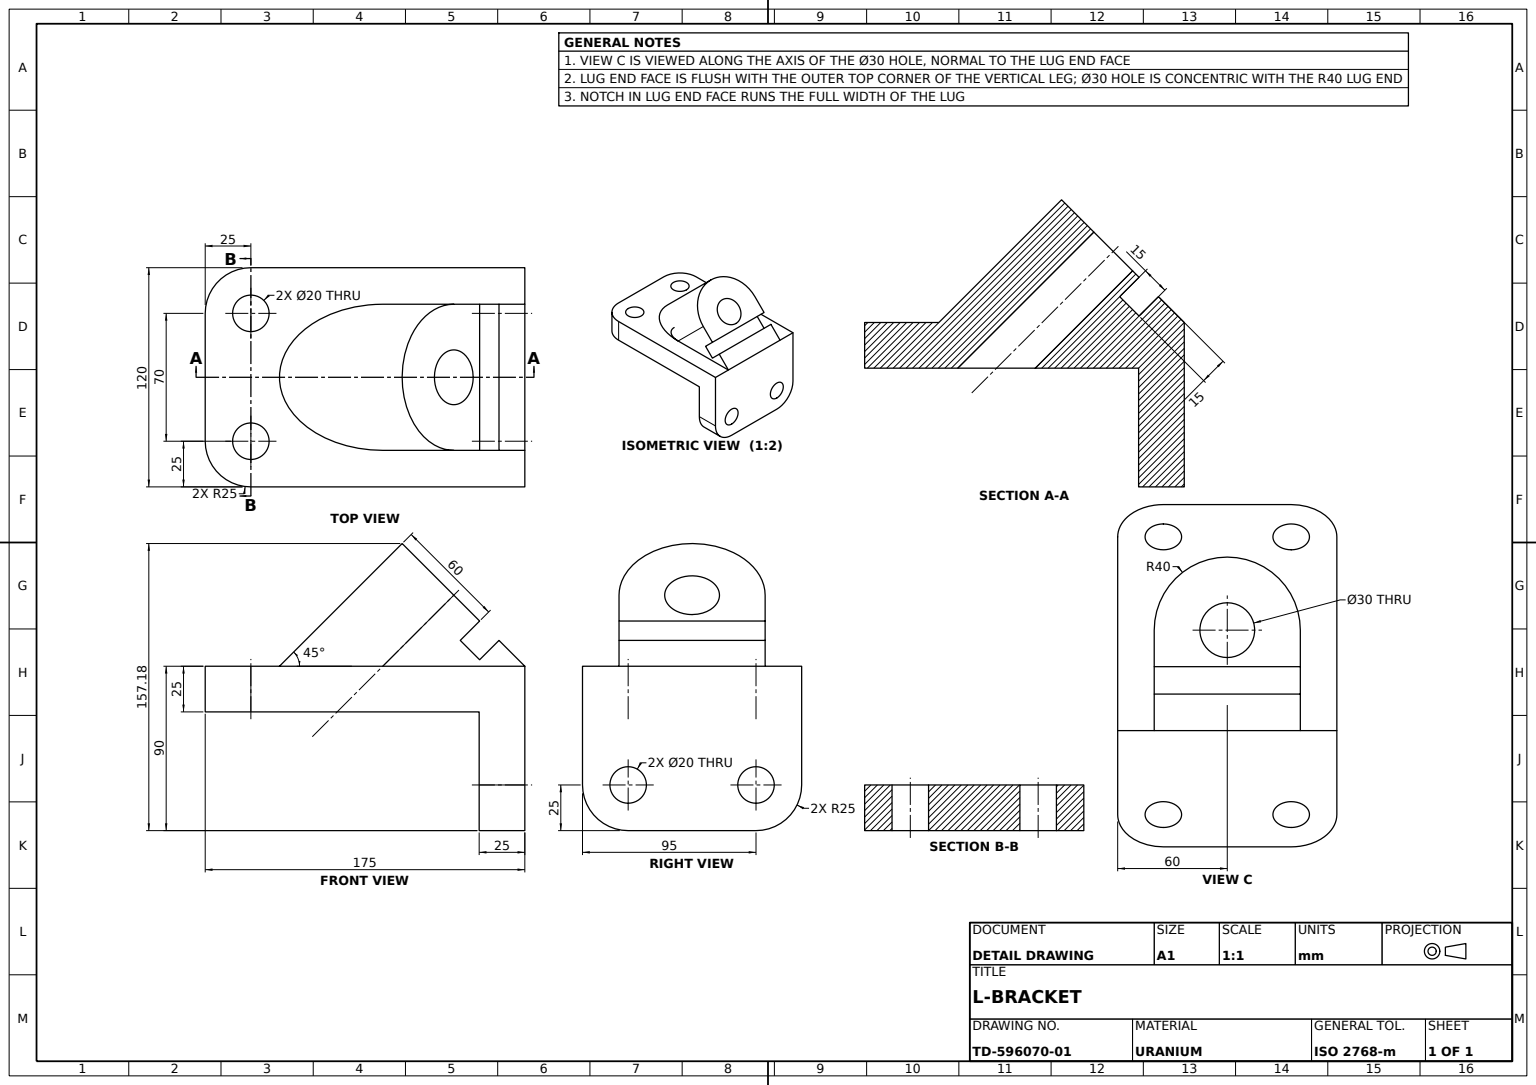
ISO-10303-21;
HEADER;
FILE_DESCRIPTION((''),'2;1');
FILE_NAME('','',(''),(''),'','','');
FILE_SCHEMA(('AUTOMOTIVE_DESIGN'));
ENDSEC;
DATA;
#1=APPLICATION_CONTEXT('');
#2=PRODUCT_CONTEXT('',#1,'mechanical');
#3=PRODUCT('','','',(#2));
#4=PRODUCT_DEFINITION_FORMATION('','',#3);
#5=PRODUCT_DEFINITION_CONTEXT('',#1,'design');
#6=PRODUCT_DEFINITION('','',#4,#5);
#7=PRODUCT_DEFINITION_SHAPE('','',#6);
#8=(LENGTH_UNIT()NAMED_UNIT(*)SI_UNIT(.MILLI.,.METRE.));
#9=(NAMED_UNIT(*)PLANE_ANGLE_UNIT()SI_UNIT($,.RADIAN.));
#10=(NAMED_UNIT(*)SI_UNIT($,.STERADIAN.)SOLID_ANGLE_UNIT());
#11=UNCERTAINTY_MEASURE_WITH_UNIT(LENGTH_MEASURE(0.005),#8,'distance_accuracy_value','');
#12=(GEOMETRIC_REPRESENTATION_CONTEXT(3)GLOBAL_UNCERTAINTY_ASSIGNED_CONTEXT((#11))GLOBAL_UNIT_ASSIGNED_CONTEXT((#8,#9,#10))REPRESENTATION_CONTEXT('',''));
#13=CARTESIAN_POINT('',(-81.568542,0.,-25.));
#14=VERTEX_POINT('',#13);
#15=CARTESIAN_POINT('',(-102.781746,0.,-25.));
#16=DIRECTION('',(0.,0.,1.));
#17=DIRECTION('',(1.,0.,0.));
#18=AXIS2_PLACEMENT_3D('',#15,#16,#17);
#19=ELLIPSE('',#18,21.213203,15.);
#20=EDGE_CURVE('',#14,#14,#19,.T.);
#21=ORIENTED_EDGE('',*,*,#20,.T.);
#22=EDGE_LOOP('',(#21));
#23=FACE_BOUND('',#22,.T.);
#24=CARTESIAN_POINT('',(-140.,-35.,-25.));
#25=VERTEX_POINT('',#24);
#26=CARTESIAN_POINT('',(-150.,-35.,-25.));
#27=AXIS2_PLACEMENT_3D('',#26,#16,#17);
#28=CIRCLE('',#27,10.);
#29=EDGE_CURVE('',#25,#25,#28,.T.);
#30=ORIENTED_EDGE('',*,*,#29,.T.);
#31=EDGE_LOOP('',(#30));
#32=FACE_BOUND('',#31,.T.);
#33=CARTESIAN_POINT('',(-175.,-35.,-25.));
#34=VERTEX_POINT('',#33);
#35=CARTESIAN_POINT('',(-175.,35.,-25.));
#36=VERTEX_POINT('',#35);
#37=CARTESIAN_POINT('',(-175.,0.,-25.));
#38=DIRECTION('',(0.,1.,0.));
#39=VECTOR('',#38,1000.);
#40=LINE('',#37,#39);
#41=EDGE_CURVE('',#34,#36,#40,.T.);
#42=ORIENTED_EDGE('',*,*,#41,.T.);
#43=CARTESIAN_POINT('',(-150.,60.,-25.));
#44=VERTEX_POINT('',#43);
#45=CARTESIAN_POINT('',(-150.,35.,-25.));
#46=AXIS2_PLACEMENT_3D('',#45,#16,#17);
#47=CIRCLE('',#46,25.);
#48=EDGE_CURVE('',#44,#36,#47,.T.);
#49=ORIENTED_EDGE('',*,*,#48,.F.);
#50=CARTESIAN_POINT('',(-25.,60.,-25.));
#51=VERTEX_POINT('',#50);
#52=CARTESIAN_POINT('',(0.,60.,-25.));
#53=VECTOR('',#17,1000.);
#54=LINE('',#52,#53);
#55=EDGE_CURVE('',#44,#51,#54,.T.);
#56=ORIENTED_EDGE('',*,*,#55,.T.);
#57=CARTESIAN_POINT('',(-25.,-60.,-25.));
#58=VERTEX_POINT('',#57);
#59=CARTESIAN_POINT('',(-25.,0.,-25.));
#60=LINE('',#59,#39);
#61=EDGE_CURVE('',#58,#51,#60,.T.);
#62=ORIENTED_EDGE('',*,*,#61,.F.);
#63=CARTESIAN_POINT('',(-150.,-60.,-25.));
#64=VERTEX_POINT('',#63);
#65=CARTESIAN_POINT('',(0.,-60.,-25.));
#66=LINE('',#65,#53);
#67=EDGE_CURVE('',#64,#58,#66,.T.);
#68=ORIENTED_EDGE('',*,*,#67,.F.);
#69=CIRCLE('',#27,25.);
#70=EDGE_CURVE('',#34,#64,#69,.T.);
#71=ORIENTED_EDGE('',*,*,#70,.F.);
#72=EDGE_LOOP('',(#42,#49,#56,#62,#68,#71));
#73=FACE_BOUND('',#72,.T.);
#74=CARTESIAN_POINT('',(-140.,35.,-25.));
#75=VERTEX_POINT('',#74);
#76=CIRCLE('',#46,10.);
#77=EDGE_CURVE('',#75,#75,#76,.T.);
#78=ORIENTED_EDGE('',*,*,#77,.T.);
#79=EDGE_LOOP('',(#78));
#80=FACE_BOUND('',#79,.T.);
#81=AXIS2_PLACEMENT_3D('',#37,#16,#17);
#82=PLANE('',#81);
#83=ADVANCED_FACE('',(#23,#32,#73,#80),#82,.F.);
#84=ORIENTED_EDGE('',*,*,#20,.F.);
#85=EDGE_LOOP('',(#84));
#86=FACE_BOUND('',#85,.T.);
#87=CARTESIAN_POINT('',(-28.284271,0.,28.284271));
#88=VERTEX_POINT('',#87);
#89=CARTESIAN_POINT('',(-38.890873,0.,38.890873));
#90=DIRECTION('',(0.707106781,0.,0.707106781));
#91=DIRECTION('',(0.707106781,0.,-0.707106781));
#92=AXIS2_PLACEMENT_3D('',#89,#90,#91);
#93=CIRCLE('',#92,15.);
#94=EDGE_CURVE('',#88,#88,#93,.T.);
#95=ORIENTED_EDGE('',*,*,#94,.T.);
#96=EDGE_LOOP('',(#95));
#97=FACE_BOUND('',#96,.T.);
#98=CARTESIAN_POINT('',(-116.261028,0.,-38.479282));
#99=AXIS2_PLACEMENT_3D('',#98,#90,#38);
#100=CYLINDRICAL_SURFACE('',#99,15.);
#101=ADVANCED_FACE('',(#86,#97),#100,.F.);
#102=CARTESIAN_POINT('',(-38.890873,40.,38.890873));
#103=VERTEX_POINT('',#102);
#104=CARTESIAN_POINT('',(-24.748737,40.,24.748737));
#105=VERTEX_POINT('',#104);
#106=VECTOR('',#91,1000.);
#107=LINE('',#102,#106);
#108=EDGE_CURVE('',#103,#105,#107,.T.);
#109=ORIENTED_EDGE('',*,*,#108,.T.);
#110=CARTESIAN_POINT('',(-35.355339,40.,14.142136));
#111=VERTEX_POINT('',#110);
#112=DIRECTION('',(-0.707106781,0.,-0.707106781));
#113=VECTOR('',#112,1000.);
#114=LINE('',#104,#113);
#115=EDGE_CURVE('',#105,#111,#114,.T.);
#116=ORIENTED_EDGE('',*,*,#115,.T.);
#117=CARTESIAN_POINT('',(-24.748737,40.,3.535534));
#118=VERTEX_POINT('',#117);
#119=CARTESIAN_POINT('',(-10.606602,40.,-10.606602));
#120=DIRECTION('',(-0.707106781,0.,0.707106781));
#121=VECTOR('',#120,1000.);
#122=LINE('',#119,#121);
#123=EDGE_CURVE('',#118,#111,#122,.T.);
#124=ORIENTED_EDGE('',*,*,#123,.F.);
#125=CARTESIAN_POINT('',(-14.142136,40.,14.142136));
#126=VERTEX_POINT('',#125);
#127=LINE('',#125,#113);
#128=EDGE_CURVE('',#126,#118,#127,.T.);
#129=ORIENTED_EDGE('',*,*,#128,.F.);
#130=CARTESIAN_POINT('',(0.,40.,0.));
#131=VERTEX_POINT('',#130);
#132=EDGE_CURVE('',#126,#131,#107,.T.);
#133=ORIENTED_EDGE('',*,*,#132,.T.);
#134=CARTESIAN_POINT('',(-77.781746,40.,0.));
#135=VERTEX_POINT('',#134);
#136=CARTESIAN_POINT('',(-38.890873,40.,0.));
#137=DIRECTION('',(-1.,0.,0.));
#138=VECTOR('',#137,1000.);
#139=LINE('',#136,#138);
#140=EDGE_CURVE('',#131,#135,#139,.T.);
#141=ORIENTED_EDGE('',*,*,#140,.T.);
#142=CARTESIAN_POINT('',(-139.241998,40.,-61.460253));
#143=VECTOR('',#90,1000.);
#144=LINE('',#142,#143);
#145=EDGE_CURVE('',#103,#135,#144,.F.);
#146=ORIENTED_EDGE('',*,*,#145,.F.);
#147=EDGE_LOOP('',(#109,#116,#124,#129,#133,#141,#146));
#148=FACE_BOUND('',#147,.T.);
#149=AXIS2_PLACEMENT_3D('',#102,#38,#91);
#150=PLANE('',#149);
#151=ADVANCED_FACE('',(#148),#150,.T.);
#152=CARTESIAN_POINT('',(-77.781746,-40.,0.));
#153=VERTEX_POINT('',#152);
#154=CARTESIAN_POINT('',(-77.781746,0.,0.));
#155=DIRECTION('',(0.,0.,-1.));
#156=AXIS2_PLACEMENT_3D('',#154,#155,#17);
#157=ELLIPSE('',#156,56.568542,40.);
#158=EDGE_CURVE('',#135,#153,#157,.F.);
#159=ORIENTED_EDGE('',*,*,#158,.F.);
#160=ORIENTED_EDGE('',*,*,#140,.F.);
#161=CARTESIAN_POINT('',(0.,60.,0.));
#162=VERTEX_POINT('',#161);
#163=CARTESIAN_POINT('',(0.,0.,0.));
#164=LINE('',#163,#39);
#165=EDGE_CURVE('',#131,#162,#164,.T.);
#166=ORIENTED_EDGE('',*,*,#165,.T.);
#167=CARTESIAN_POINT('',(-150.,60.,0.));
#168=VERTEX_POINT('',#167);
#169=LINE('',#161,#138);
#170=EDGE_CURVE('',#162,#168,#169,.T.);
#171=ORIENTED_EDGE('',*,*,#170,.T.);
#172=CARTESIAN_POINT('',(-175.,35.,0.));
#173=VERTEX_POINT('',#172);
#174=CARTESIAN_POINT('',(-150.,35.,0.));
#175=AXIS2_PLACEMENT_3D('',#174,#155,#137);
#176=CIRCLE('',#175,25.);
#177=EDGE_CURVE('',#173,#168,#176,.T.);
#178=ORIENTED_EDGE('',*,*,#177,.F.);
#179=CARTESIAN_POINT('',(-175.,-35.,0.));
#180=VERTEX_POINT('',#179);
#181=CARTESIAN_POINT('',(-175.,0.,0.));
#182=LINE('',#181,#39);
#183=EDGE_CURVE('',#180,#173,#182,.T.);
#184=ORIENTED_EDGE('',*,*,#183,.F.);
#185=CARTESIAN_POINT('',(-150.,-60.,0.));
#186=VERTEX_POINT('',#185);
#187=CARTESIAN_POINT('',(-150.,-35.,0.));
#188=AXIS2_PLACEMENT_3D('',#187,#155,#137);
#189=CIRCLE('',#188,25.);
#190=EDGE_CURVE('',#186,#180,#189,.T.);
#191=ORIENTED_EDGE('',*,*,#190,.F.);
#192=CARTESIAN_POINT('',(0.,-60.,0.));
#193=VERTEX_POINT('',#192);
#194=LINE('',#192,#138);
#195=EDGE_CURVE('',#193,#186,#194,.T.);
#196=ORIENTED_EDGE('',*,*,#195,.F.);
#197=CARTESIAN_POINT('',(0.,-40.,0.));
#198=VERTEX_POINT('',#197);
#199=EDGE_CURVE('',#193,#198,#164,.T.);
#200=ORIENTED_EDGE('',*,*,#199,.T.);
#201=LINE('',#197,#138);
#202=EDGE_CURVE('',#198,#153,#201,.T.);
#203=ORIENTED_EDGE('',*,*,#202,.T.);
#204=EDGE_LOOP('',(#159,#160,#166,#171,#178,#184,#191,#196,#200,#203));
#205=FACE_BOUND('',#204,.T.);
#206=CARTESIAN_POINT('',(-160.,-35.,0.));
#207=VERTEX_POINT('',#206);
#208=CIRCLE('',#188,10.);
#209=EDGE_CURVE('',#207,#207,#208,.F.);
#210=ORIENTED_EDGE('',*,*,#209,.F.);
#211=EDGE_LOOP('',(#210));
#212=FACE_BOUND('',#211,.T.);
#213=CARTESIAN_POINT('',(-160.,35.,0.));
#214=VERTEX_POINT('',#213);
#215=CIRCLE('',#175,10.);
#216=EDGE_CURVE('',#214,#214,#215,.F.);
#217=ORIENTED_EDGE('',*,*,#216,.F.);
#218=EDGE_LOOP('',(#217));
#219=FACE_BOUND('',#218,.T.);
#220=AXIS2_PLACEMENT_3D('',#163,#155,#137);
#221=PLANE('',#220);
#222=ADVANCED_FACE('',(#205,#212,#219),#221,.F.);
#223=ORIENTED_EDGE('',*,*,#132,.F.);
#224=CARTESIAN_POINT('',(-14.142136,-40.,14.142136));
#225=VERTEX_POINT('',#224);
#226=LINE('',#224,#39);
#227=EDGE_CURVE('',#225,#126,#226,.T.);
#228=ORIENTED_EDGE('',*,*,#227,.F.);
#229=LINE('',#197,#121);
#230=EDGE_CURVE('',#198,#225,#229,.T.);
#231=ORIENTED_EDGE('',*,*,#230,.F.);
#232=DIRECTION('',(0.,-1.,0.));
#233=VECTOR('',#232,1000.);
#234=LINE('',#163,#233);
#235=EDGE_CURVE('',#131,#198,#234,.T.);
#236=ORIENTED_EDGE('',*,*,#235,.F.);
#237=EDGE_LOOP('',(#223,#228,#231,#236));
#238=FACE_BOUND('',#237,.T.);
#239=AXIS2_PLACEMENT_3D('',#163,#90,#38);
#240=PLANE('',#239);
#241=ADVANCED_FACE('',(#238),#240,.T.);
#242=CARTESIAN_POINT('',(-24.748737,-40.,24.748737));
#243=VERTEX_POINT('',#242);
#244=CARTESIAN_POINT('',(-35.355339,-40.,14.142136));
#245=VERTEX_POINT('',#244);
#246=LINE('',#242,#113);
#247=EDGE_CURVE('',#243,#245,#246,.T.);
#248=ORIENTED_EDGE('',*,*,#247,.T.);
#249=LINE('',#110,#233);
#250=EDGE_CURVE('',#111,#245,#249,.T.);
#251=ORIENTED_EDGE('',*,*,#250,.F.);
#252=ORIENTED_EDGE('',*,*,#115,.F.);
#253=LINE('',#104,#233);
#254=EDGE_CURVE('',#105,#243,#253,.T.);
#255=ORIENTED_EDGE('',*,*,#254,.T.);
#256=EDGE_LOOP('',(#248,#251,#252,#255));
#257=FACE_BOUND('',#256,.T.);
#258=AXIS2_PLACEMENT_3D('',#104,#91,#232);
#259=PLANE('',#258);
#260=ADVANCED_FACE('',(#257),#259,.T.);
#261=CARTESIAN_POINT('',(0.,-35.,-55.));
#262=VERTEX_POINT('',#261);
#263=CARTESIAN_POINT('',(0.,-35.,-65.));
#264=AXIS2_PLACEMENT_3D('',#263,#137,#16);
#265=CIRCLE('',#264,10.);
#266=EDGE_CURVE('',#262,#262,#265,.F.);
#267=ORIENTED_EDGE('',*,*,#266,.T.);
#268=EDGE_LOOP('',(#267));
#269=FACE_BOUND('',#268,.T.);
#270=CARTESIAN_POINT('',(-25.,-35.,-75.));
#271=VERTEX_POINT('',#270);
#272=CARTESIAN_POINT('',(-25.,-35.,-65.));
#273=AXIS2_PLACEMENT_3D('',#272,#17,#155);
#274=CIRCLE('',#273,10.);
#275=EDGE_CURVE('',#271,#271,#274,.T.);
#276=ORIENTED_EDGE('',*,*,#275,.F.);
#277=EDGE_LOOP('',(#276));
#278=FACE_BOUND('',#277,.T.);
#279=CARTESIAN_POINT('',(-88.16,-35.,-65.));
#280=AXIS2_PLACEMENT_3D('',#279,#17,#38);
#281=CYLINDRICAL_SURFACE('',#280,10.);
#282=ADVANCED_FACE('',(#269,#278),#281,.F.);
#283=CARTESIAN_POINT('',(-38.890873,-40.,38.890873));
#284=VERTEX_POINT('',#283);
#285=EDGE_CURVE('',#243,#284,#229,.T.);
#286=ORIENTED_EDGE('',*,*,#285,.F.);
#287=ORIENTED_EDGE('',*,*,#254,.F.);
#288=ORIENTED_EDGE('',*,*,#108,.F.);
#289=CIRCLE('',#92,40.);
#290=EDGE_CURVE('',#103,#284,#289,.T.);
#291=ORIENTED_EDGE('',*,*,#290,.T.);
#292=EDGE_LOOP('',(#286,#287,#288,#291));
#293=FACE_BOUND('',#292,.T.);
#294=ORIENTED_EDGE('',*,*,#94,.F.);
#295=EDGE_LOOP('',(#294));
#296=FACE_BOUND('',#295,.T.);
#297=ADVANCED_FACE('',(#293,#296),#240,.T.);
#298=ORIENTED_EDGE('',*,*,#266,.F.);
#299=EDGE_LOOP('',(#298));
#300=FACE_BOUND('',#299,.T.);
#301=ORIENTED_EDGE('',*,*,#165,.F.);
#302=ORIENTED_EDGE('',*,*,#235,.T.);
#303=ORIENTED_EDGE('',*,*,#199,.F.);
#304=CARTESIAN_POINT('',(0.,-60.,-65.));
#305=VERTEX_POINT('',#304);
#306=VECTOR('',#16,1000.);
#307=LINE('',#192,#306);
#308=EDGE_CURVE('',#305,#193,#307,.T.);
#309=ORIENTED_EDGE('',*,*,#308,.F.);
#310=CARTESIAN_POINT('',(0.,-35.,-90.));
#311=VERTEX_POINT('',#310);
#312=CIRCLE('',#264,25.);
#313=EDGE_CURVE('',#311,#305,#312,.T.);
#314=ORIENTED_EDGE('',*,*,#313,.F.);
#315=CARTESIAN_POINT('',(0.,35.,-90.));
#316=VERTEX_POINT('',#315);
#317=CARTESIAN_POINT('',(0.,0.,-90.));
#318=LINE('',#317,#39);
#319=EDGE_CURVE('',#311,#316,#318,.T.);
#320=ORIENTED_EDGE('',*,*,#319,.T.);
#321=CARTESIAN_POINT('',(0.,60.,-65.));
#322=VERTEX_POINT('',#321);
#323=CARTESIAN_POINT('',(0.,35.,-65.));
#324=AXIS2_PLACEMENT_3D('',#323,#137,#16);
#325=CIRCLE('',#324,25.);
#326=EDGE_CURVE('',#322,#316,#325,.T.);
#327=ORIENTED_EDGE('',*,*,#326,.F.);
#328=LINE('',#161,#306);
#329=EDGE_CURVE('',#322,#162,#328,.T.);
#330=ORIENTED_EDGE('',*,*,#329,.T.);
#331=EDGE_LOOP('',(#301,#302,#303,#309,#314,#320,#327,#330));
#332=FACE_BOUND('',#331,.T.);
#333=CARTESIAN_POINT('',(0.,35.,-55.));
#334=VERTEX_POINT('',#333);
#335=CIRCLE('',#324,10.);
#336=EDGE_CURVE('',#334,#334,#335,.F.);
#337=ORIENTED_EDGE('',*,*,#336,.F.);
#338=EDGE_LOOP('',(#337));
#339=FACE_BOUND('',#338,.T.);
#340=AXIS2_PLACEMENT_3D('',#317,#137,#16);
#341=PLANE('',#340);
#342=ADVANCED_FACE('',(#300,#332,#339),#341,.F.);
#343=ORIENTED_EDGE('',*,*,#308,.T.);
#344=ORIENTED_EDGE('',*,*,#195,.T.);
#345=CARTESIAN_POINT('',(-150.,-60.,-32.5));
#346=VECTOR('',#155,1000.);
#347=LINE('',#345,#346);
#348=EDGE_CURVE('',#186,#64,#347,.T.);
#349=ORIENTED_EDGE('',*,*,#348,.T.);
#350=ORIENTED_EDGE('',*,*,#67,.T.);
#351=CARTESIAN_POINT('',(-25.,-60.,-65.));
#352=VERTEX_POINT('',#351);
#353=CARTESIAN_POINT('',(-25.,-60.,0.));
#354=LINE('',#353,#346);
#355=EDGE_CURVE('',#58,#352,#354,.T.);
#356=ORIENTED_EDGE('',*,*,#355,.T.);
#357=CARTESIAN_POINT('',(-87.5,-60.,-65.));
#358=LINE('',#357,#53);
#359=EDGE_CURVE('',#352,#305,#358,.T.);
#360=ORIENTED_EDGE('',*,*,#359,.T.);
#361=EDGE_LOOP('',(#343,#344,#349,#350,#356,#360));
#362=FACE_BOUND('',#361,.T.);
#363=AXIS2_PLACEMENT_3D('',#192,#38,#137);
#364=PLANE('',#363);
#365=ADVANCED_FACE('',(#362),#364,.F.);
#366=CARTESIAN_POINT('',(-25.,-35.,-90.));
#367=VERTEX_POINT('',#366);
#368=CARTESIAN_POINT('',(-25.,35.,-90.));
#369=VERTEX_POINT('',#368);
#370=CARTESIAN_POINT('',(-25.,0.,-90.));
#371=LINE('',#370,#39);
#372=EDGE_CURVE('',#367,#369,#371,.T.);
#373=ORIENTED_EDGE('',*,*,#372,.T.);
#374=CARTESIAN_POINT('',(-87.5,35.,-90.));
#375=LINE('',#374,#53);
#376=EDGE_CURVE('',#369,#316,#375,.T.);
#377=ORIENTED_EDGE('',*,*,#376,.T.);
#378=ORIENTED_EDGE('',*,*,#319,.F.);
#379=CARTESIAN_POINT('',(-87.5,-35.,-90.));
#380=LINE('',#379,#53);
#381=EDGE_CURVE('',#367,#311,#380,.T.);
#382=ORIENTED_EDGE('',*,*,#381,.F.);
#383=EDGE_LOOP('',(#373,#377,#378,#382));
#384=FACE_BOUND('',#383,.T.);
#385=AXIS2_PLACEMENT_3D('',#370,#16,#17);
#386=PLANE('',#385);
#387=ADVANCED_FACE('',(#384),#386,.F.);
#388=CARTESIAN_POINT('',(-175.,35.,-32.5));
#389=LINE('',#388,#346);
#390=EDGE_CURVE('',#173,#36,#389,.T.);
#391=ORIENTED_EDGE('',*,*,#390,.T.);
#392=ORIENTED_EDGE('',*,*,#41,.F.);
#393=CARTESIAN_POINT('',(-175.,-35.,-32.5));
#394=LINE('',#393,#346);
#395=EDGE_CURVE('',#180,#34,#394,.T.);
#396=ORIENTED_EDGE('',*,*,#395,.F.);
#397=ORIENTED_EDGE('',*,*,#183,.T.);
#398=EDGE_LOOP('',(#391,#392,#396,#397));
#399=FACE_BOUND('',#398,.T.);
#400=AXIS2_PLACEMENT_3D('',#181,#17,#155);
#401=PLANE('',#400);
#402=ADVANCED_FACE('',(#399),#401,.F.);
#403=ORIENTED_EDGE('',*,*,#313,.T.);
#404=ORIENTED_EDGE('',*,*,#359,.F.);
#405=CIRCLE('',#273,25.);
#406=EDGE_CURVE('',#352,#367,#405,.T.);
#407=ORIENTED_EDGE('',*,*,#406,.T.);
#408=ORIENTED_EDGE('',*,*,#381,.T.);
#409=EDGE_LOOP('',(#403,#404,#407,#408));
#410=FACE_BOUND('',#409,.T.);
#411=CARTESIAN_POINT('',(-87.5,-35.,-65.));
#412=AXIS2_PLACEMENT_3D('',#411,#17,#232);
#413=CYLINDRICAL_SURFACE('',#412,25.);
#414=ADVANCED_FACE('',(#410),#413,.T.);
#415=ORIENTED_EDGE('',*,*,#290,.F.);
#416=ORIENTED_EDGE('',*,*,#145,.T.);
#417=ORIENTED_EDGE('',*,*,#158,.T.);
#418=CARTESIAN_POINT('',(-139.241998,-40.,-61.460253));
#419=LINE('',#418,#143);
#420=EDGE_CURVE('',#284,#153,#419,.F.);
#421=ORIENTED_EDGE('',*,*,#420,.F.);
#422=EDGE_LOOP('',(#415,#416,#417,#421));
#423=FACE_BOUND('',#422,.T.);
#424=CARTESIAN_POINT('',(-139.241998,0.,-61.460253));
#425=AXIS2_PLACEMENT_3D('',#424,#90,#38);
#426=CYLINDRICAL_SURFACE('',#425,40.);
#427=ADVANCED_FACE('',(#423),#426,.T.);
#428=ORIENTED_EDGE('',*,*,#420,.T.);
#429=ORIENTED_EDGE('',*,*,#202,.F.);
#430=ORIENTED_EDGE('',*,*,#230,.T.);
#431=CARTESIAN_POINT('',(-24.748737,-40.,3.535534));
#432=VERTEX_POINT('',#431);
#433=LINE('',#224,#113);
#434=EDGE_CURVE('',#225,#432,#433,.T.);
#435=ORIENTED_EDGE('',*,*,#434,.T.);
#436=CARTESIAN_POINT('',(-10.606602,-40.,-10.606602));
#437=LINE('',#436,#106);
#438=EDGE_CURVE('',#245,#432,#437,.T.);
#439=ORIENTED_EDGE('',*,*,#438,.F.);
#440=ORIENTED_EDGE('',*,*,#247,.F.);
#441=ORIENTED_EDGE('',*,*,#285,.T.);
#442=EDGE_LOOP('',(#428,#429,#430,#435,#439,#440,#441));
#443=FACE_BOUND('',#442,.T.);
#444=AXIS2_PLACEMENT_3D('',#197,#232,#120);
#445=PLANE('',#444);
#446=ADVANCED_FACE('',(#443),#445,.T.);
#447=ORIENTED_EDGE('',*,*,#227,.T.);
#448=ORIENTED_EDGE('',*,*,#128,.T.);
#449=LINE('',#431,#39);
#450=EDGE_CURVE('',#432,#118,#449,.T.);
#451=ORIENTED_EDGE('',*,*,#450,.F.);
#452=ORIENTED_EDGE('',*,*,#434,.F.);
#453=EDGE_LOOP('',(#447,#448,#451,#452));
#454=FACE_BOUND('',#453,.T.);
#455=AXIS2_PLACEMENT_3D('',#224,#120,#38);
#456=PLANE('',#455);
#457=ADVANCED_FACE('',(#454),#456,.T.);
#458=ORIENTED_EDGE('',*,*,#348,.F.);
#459=ORIENTED_EDGE('',*,*,#190,.T.);
#460=ORIENTED_EDGE('',*,*,#395,.T.);
#461=ORIENTED_EDGE('',*,*,#70,.T.);
#462=EDGE_LOOP('',(#458,#459,#460,#461));
#463=FACE_BOUND('',#462,.T.);
#464=CARTESIAN_POINT('',(-150.,-35.,-32.5));
#465=AXIS2_PLACEMENT_3D('',#464,#155,#232);
#466=CYLINDRICAL_SURFACE('',#465,25.);
#467=ADVANCED_FACE('',(#463),#466,.T.);
#468=ORIENTED_EDGE('',*,*,#450,.T.);
#469=ORIENTED_EDGE('',*,*,#123,.T.);
#470=ORIENTED_EDGE('',*,*,#250,.T.);
#471=ORIENTED_EDGE('',*,*,#438,.T.);
#472=EDGE_LOOP('',(#468,#469,#470,#471));
#473=FACE_BOUND('',#472,.T.);
#474=CARTESIAN_POINT('',(-10.606602,0.,-10.606602));
#475=AXIS2_PLACEMENT_3D('',#474,#90,#38);
#476=PLANE('',#475);
#477=ADVANCED_FACE('',(#473),#476,.T.);
#478=ORIENTED_EDGE('',*,*,#177,.T.);
#479=CARTESIAN_POINT('',(-150.,60.,-32.5));
#480=LINE('',#479,#346);
#481=EDGE_CURVE('',#168,#44,#480,.T.);
#482=ORIENTED_EDGE('',*,*,#481,.T.);
#483=ORIENTED_EDGE('',*,*,#48,.T.);
#484=ORIENTED_EDGE('',*,*,#390,.F.);
#485=EDGE_LOOP('',(#478,#482,#483,#484));
#486=FACE_BOUND('',#485,.T.);
#487=CARTESIAN_POINT('',(-150.,35.,-32.5));
#488=AXIS2_PLACEMENT_3D('',#487,#155,#137);
#489=CYLINDRICAL_SURFACE('',#488,25.);
#490=ADVANCED_FACE('',(#486),#489,.T.);
#491=ORIENTED_EDGE('',*,*,#55,.F.);
#492=ORIENTED_EDGE('',*,*,#481,.F.);
#493=ORIENTED_EDGE('',*,*,#170,.F.);
#494=ORIENTED_EDGE('',*,*,#329,.F.);
#495=CARTESIAN_POINT('',(-25.,60.,-65.));
#496=VERTEX_POINT('',#495);
#497=CARTESIAN_POINT('',(-87.5,60.,-65.));
#498=LINE('',#497,#53);
#499=EDGE_CURVE('',#496,#322,#498,.T.);
#500=ORIENTED_EDGE('',*,*,#499,.F.);
#501=CARTESIAN_POINT('',(-25.,60.,0.));
#502=LINE('',#501,#346);
#503=EDGE_CURVE('',#51,#496,#502,.T.);
#504=ORIENTED_EDGE('',*,*,#503,.F.);
#505=EDGE_LOOP('',(#491,#492,#493,#494,#500,#504));
#506=FACE_BOUND('',#505,.T.);
#507=AXIS2_PLACEMENT_3D('',#161,#38,#137);
#508=PLANE('',#507);
#509=ADVANCED_FACE('',(#506),#508,.T.);
#510=ORIENTED_EDGE('',*,*,#275,.T.);
#511=EDGE_LOOP('',(#510));
#512=FACE_BOUND('',#511,.T.);
#513=ORIENTED_EDGE('',*,*,#503,.T.);
#514=CARTESIAN_POINT('',(-25.,35.,-65.));
#515=AXIS2_PLACEMENT_3D('',#514,#17,#155);
#516=CIRCLE('',#515,25.);
#517=EDGE_CURVE('',#369,#496,#516,.T.);
#518=ORIENTED_EDGE('',*,*,#517,.F.);
#519=ORIENTED_EDGE('',*,*,#372,.F.);
#520=ORIENTED_EDGE('',*,*,#406,.F.);
#521=ORIENTED_EDGE('',*,*,#355,.F.);
#522=ORIENTED_EDGE('',*,*,#61,.T.);
#523=EDGE_LOOP('',(#513,#518,#519,#520,#521,#522));
#524=FACE_BOUND('',#523,.T.);
#525=CARTESIAN_POINT('',(-25.,35.,-75.));
#526=VERTEX_POINT('',#525);
#527=CIRCLE('',#515,10.);
#528=EDGE_CURVE('',#526,#526,#527,.T.);
#529=ORIENTED_EDGE('',*,*,#528,.T.);
#530=EDGE_LOOP('',(#529));
#531=FACE_BOUND('',#530,.T.);
#532=AXIS2_PLACEMENT_3D('',#59,#17,#155);
#533=PLANE('',#532);
#534=ADVANCED_FACE('',(#512,#524,#531),#533,.F.);
#535=ORIENTED_EDGE('',*,*,#216,.T.);
#536=EDGE_LOOP('',(#535));
#537=FACE_BOUND('',#536,.T.);
#538=ORIENTED_EDGE('',*,*,#77,.F.);
#539=EDGE_LOOP('',(#538));
#540=FACE_BOUND('',#539,.T.);
#541=CARTESIAN_POINT('',(-150.,35.,-45.66));
#542=AXIS2_PLACEMENT_3D('',#541,#16,#17);
#543=CYLINDRICAL_SURFACE('',#542,10.);
#544=ADVANCED_FACE('',(#537,#540),#543,.F.);
#545=ORIENTED_EDGE('',*,*,#517,.T.);
#546=ORIENTED_EDGE('',*,*,#499,.T.);
#547=ORIENTED_EDGE('',*,*,#326,.T.);
#548=ORIENTED_EDGE('',*,*,#376,.F.);
#549=EDGE_LOOP('',(#545,#546,#547,#548));
#550=FACE_BOUND('',#549,.T.);
#551=CARTESIAN_POINT('',(-87.5,35.,-65.));
#552=AXIS2_PLACEMENT_3D('',#551,#17,#155);
#553=CYLINDRICAL_SURFACE('',#552,25.);
#554=ADVANCED_FACE('',(#550),#553,.T.);
#555=ORIENTED_EDGE('',*,*,#336,.T.);
#556=EDGE_LOOP('',(#555));
#557=FACE_BOUND('',#556,.T.);
#558=ORIENTED_EDGE('',*,*,#528,.F.);
#559=EDGE_LOOP('',(#558));
#560=FACE_BOUND('',#559,.T.);
#561=CARTESIAN_POINT('',(-88.16,35.,-65.));
#562=AXIS2_PLACEMENT_3D('',#561,#17,#38);
#563=CYLINDRICAL_SURFACE('',#562,10.);
#564=ADVANCED_FACE('',(#557,#560),#563,.F.);
#565=ORIENTED_EDGE('',*,*,#29,.F.);
#566=EDGE_LOOP('',(#565));
#567=FACE_BOUND('',#566,.T.);
#568=ORIENTED_EDGE('',*,*,#209,.T.);
#569=EDGE_LOOP('',(#568));
#570=FACE_BOUND('',#569,.T.);
#571=CARTESIAN_POINT('',(-150.,-35.,-45.66));
#572=AXIS2_PLACEMENT_3D('',#571,#16,#17);
#573=CYLINDRICAL_SURFACE('',#572,10.);
#574=ADVANCED_FACE('',(#567,#570),#573,.F.);
#575=CLOSED_SHELL('',(#83,#101,#151,#222,#241,#260,#282,#297,#342,#365,#387,#402,#414,#427,#446,#457,#467,#477,#490,#509,#534,#544,#554,#564,#574));
#576=MANIFOLD_SOLID_BREP('',#575);
#577=ADVANCED_BREP_SHAPE_REPRESENTATION('',(#576),#12);
#578=SHAPE_DEFINITION_REPRESENTATION(#7,#577);
ENDSEC;
END-ISO-10303-21;
